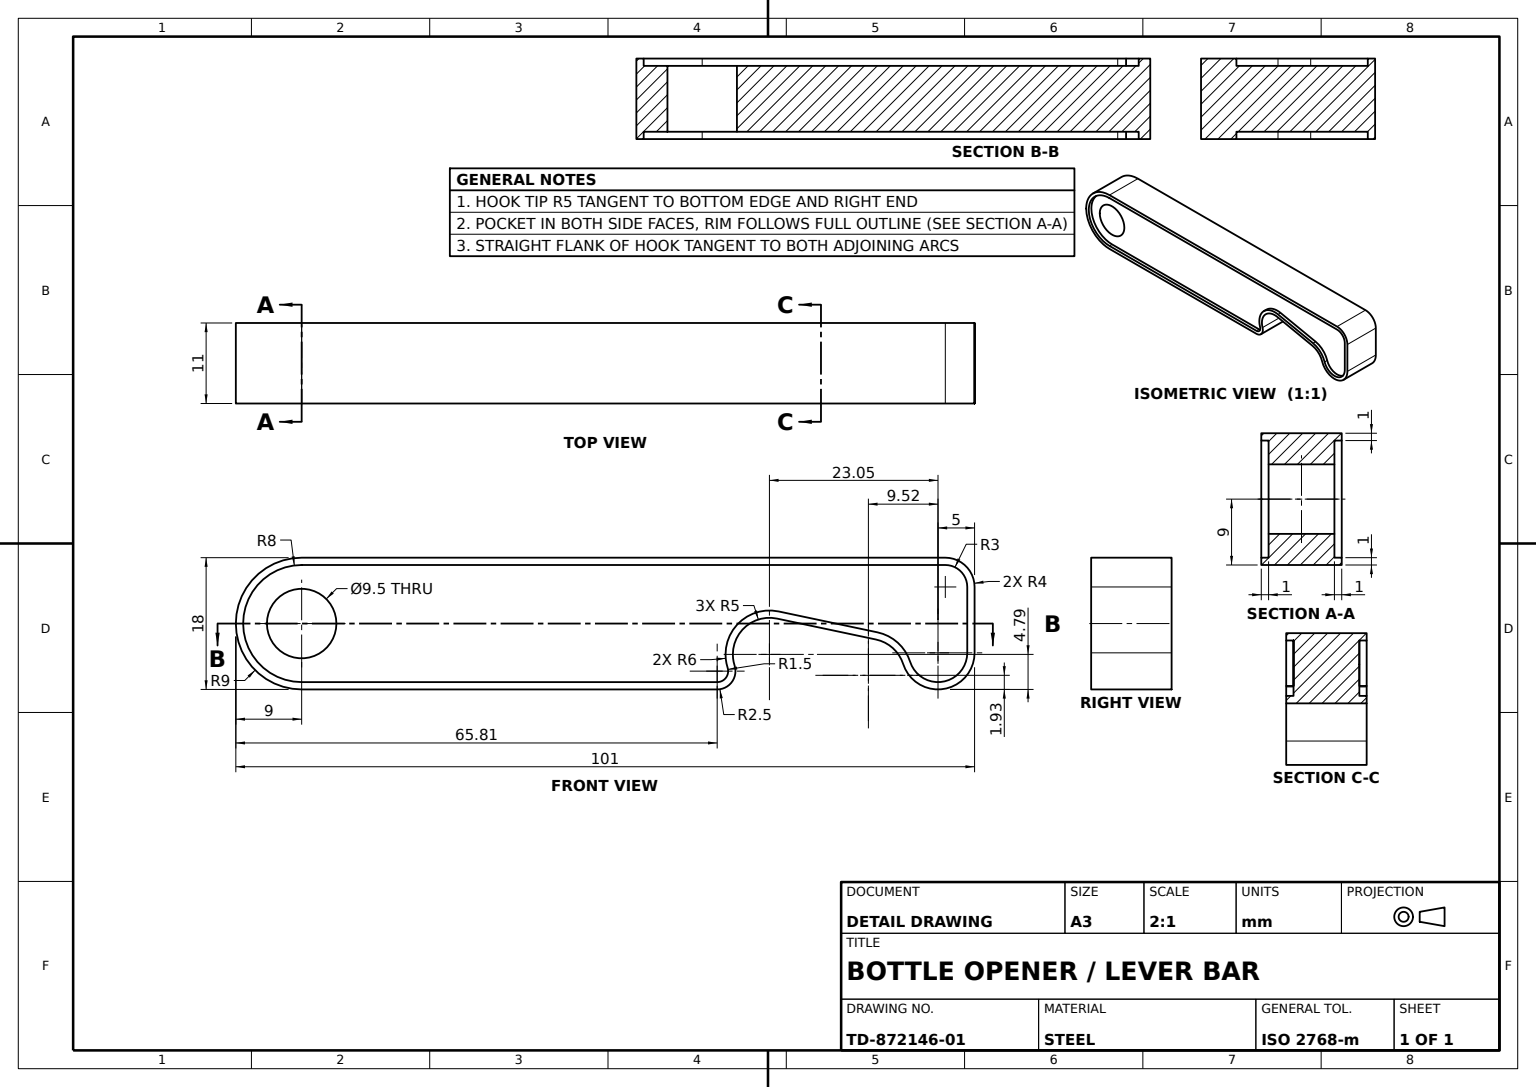
ISO-10303-21;
HEADER;
FILE_DESCRIPTION((''),'2;1');
FILE_NAME('','',(''),(''),'','','');
FILE_SCHEMA(('AUTOMOTIVE_DESIGN'));
ENDSEC;
DATA;
#1=APPLICATION_CONTEXT('');
#2=PRODUCT_CONTEXT('',#1,'mechanical');
#3=PRODUCT('','','',(#2));
#4=PRODUCT_DEFINITION_FORMATION('','',#3);
#5=PRODUCT_DEFINITION_CONTEXT('',#1,'design');
#6=PRODUCT_DEFINITION('','',#4,#5);
#7=PRODUCT_DEFINITION_SHAPE('','',#6);
#8=(LENGTH_UNIT()NAMED_UNIT(*)SI_UNIT(.MILLI.,.METRE.));
#9=(NAMED_UNIT(*)PLANE_ANGLE_UNIT()SI_UNIT($,.RADIAN.));
#10=(NAMED_UNIT(*)SI_UNIT($,.STERADIAN.)SOLID_ANGLE_UNIT());
#11=UNCERTAINTY_MEASURE_WITH_UNIT(LENGTH_MEASURE(1.E-05),#8,'distance_accuracy_value','');
#12=(GEOMETRIC_REPRESENTATION_CONTEXT(3)GLOBAL_UNCERTAINTY_ASSIGNED_CONTEXT((#11))GLOBAL_UNIT_ASSIGNED_CONTEXT((#8,#9,#10))REPRESENTATION_CONTEXT('',''));
#13=CARTESIAN_POINT('',(-9.,0.,5.5));
#14=VERTEX_POINT('',#13);
#15=CARTESIAN_POINT('',(0.,-9.,5.5));
#16=VERTEX_POINT('',#15);
#17=CARTESIAN_POINT('',(0.,0.,5.5));
#18=DIRECTION('',(0.,0.,1.));
#19=DIRECTION('',(1.,0.,0.));
#20=AXIS2_PLACEMENT_3D('',#17,#18,#19);
#21=CIRCLE('',#20,9.);
#22=EDGE_CURVE('',#14,#16,#21,.T.);
#23=ORIENTED_EDGE('',*,*,#22,.F.);
#24=CARTESIAN_POINT('',(-9.,0.,-5.5));
#25=VERTEX_POINT('',#24);
#26=CARTESIAN_POINT('',(-9.,0.,4.5));
#27=DIRECTION('',(0.,0.,-1.));
#28=VECTOR('',#27,1000.);
#29=LINE('',#26,#28);
#30=EDGE_CURVE('',#14,#25,#29,.T.);
#31=ORIENTED_EDGE('',*,*,#30,.T.);
#32=CARTESIAN_POINT('',(0.,-9.,-5.5));
#33=VERTEX_POINT('',#32);
#34=CARTESIAN_POINT('',(0.,0.,-5.5));
#35=AXIS2_PLACEMENT_3D('',#34,#18,#19);
#36=CIRCLE('',#35,9.);
#37=EDGE_CURVE('',#25,#33,#36,.T.);
#38=ORIENTED_EDGE('',*,*,#37,.T.);
#39=CARTESIAN_POINT('',(0.,-9.,4.5));
#40=LINE('',#39,#28);
#41=EDGE_CURVE('',#16,#33,#40,.T.);
#42=ORIENTED_EDGE('',*,*,#41,.F.);
#43=EDGE_LOOP('',(#23,#31,#38,#42));
#44=FACE_OUTER_BOUND('',#43,.T.);
#45=CARTESIAN_POINT('',(0.,0.,4.5));
#46=DIRECTION('',(-1.,0.,0.));
#47=AXIS2_PLACEMENT_3D('',#45,#27,#46);
#48=CYLINDRICAL_SURFACE('',#47,9.);
#49=ADVANCED_FACE('',(#44),#48,.T.);
#50=CARTESIAN_POINT('',(-4.75,0.,4.5));
#51=VERTEX_POINT('',#50);
#52=CARTESIAN_POINT('',(-4.75,0.,-4.5));
#53=VERTEX_POINT('',#52);
#54=CARTESIAN_POINT('',(-4.75,0.,11.5));
#55=LINE('',#54,#28);
#56=EDGE_CURVE('',#51,#53,#55,.T.);
#57=ORIENTED_EDGE('',*,*,#56,.F.);
#58=CARTESIAN_POINT('',(4.75,0.,4.5));
#59=VERTEX_POINT('',#58);
#60=AXIS2_PLACEMENT_3D('',#45,#18,#19);
#61=CIRCLE('',#60,4.75);
#62=EDGE_CURVE('',#51,#59,#61,.T.);
#63=ORIENTED_EDGE('',*,*,#62,.T.);
#64=CARTESIAN_POINT('',(4.75,0.,-4.5));
#65=VERTEX_POINT('',#64);
#66=CARTESIAN_POINT('',(4.75,0.,11.5));
#67=LINE('',#66,#28);
#68=EDGE_CURVE('',#59,#65,#67,.T.);
#69=ORIENTED_EDGE('',*,*,#68,.T.);
#70=CARTESIAN_POINT('',(0.,0.,-4.5));
#71=AXIS2_PLACEMENT_3D('',#70,#27,#46);
#72=CIRCLE('',#71,4.75);
#73=EDGE_CURVE('',#65,#53,#72,.T.);
#74=ORIENTED_EDGE('',*,*,#73,.T.);
#75=EDGE_LOOP('',(#57,#63,#69,#74));
#76=FACE_OUTER_BOUND('',#75,.T.);
#77=CARTESIAN_POINT('',(0.,0.,11.5));
#78=AXIS2_PLACEMENT_3D('',#77,#27,#46);
#79=CYLINDRICAL_SURFACE('',#78,4.75);
#80=ADVANCED_FACE('',(#76),#79,.F.);
#81=CARTESIAN_POINT('',(57.952121,-4.212725,5.5));
#82=VERTEX_POINT('',#81);
#83=CARTESIAN_POINT('',(57.952121,-4.212725,4.5));
#84=VERTEX_POINT('',#83);
#85=LINE('',#81,#28);
#86=EDGE_CURVE('',#82,#84,#85,.T.);
#87=ORIENTED_EDGE('',*,*,#86,.F.);
#88=CARTESIAN_POINT('',(65.192199,1.657727,5.5));
#89=VERTEX_POINT('',#88);
#90=CARTESIAN_POINT('',(63.952121,-4.212725,5.5));
#91=AXIS2_PLACEMENT_3D('',#90,#27,#19);
#92=CIRCLE('',#91,6.);
#93=EDGE_CURVE('',#82,#89,#92,.T.);
#94=ORIENTED_EDGE('',*,*,#93,.T.);
#95=CARTESIAN_POINT('',(65.192199,1.657727,4.5));
#96=VERTEX_POINT('',#95);
#97=LINE('',#88,#28);
#98=EDGE_CURVE('',#89,#96,#97,.T.);
#99=ORIENTED_EDGE('',*,*,#98,.T.);
#100=CARTESIAN_POINT('',(63.952121,-4.212725,4.5));
#101=AXIS2_PLACEMENT_3D('',#100,#27,#19);
#102=CIRCLE('',#101,6.);
#103=EDGE_CURVE('',#84,#96,#102,.T.);
#104=ORIENTED_EDGE('',*,*,#103,.F.);
#105=EDGE_LOOP('',(#87,#94,#99,#104));
#106=FACE_OUTER_BOUND('',#105,.T.);
#107=AXIS2_PLACEMENT_3D('',#90,#27,#46);
#108=CYLINDRICAL_SURFACE('',#107,6.);
#109=ADVANCED_FACE('',(#106),#108,.T.);
#110=CARTESIAN_POINT('',(83.193297,-5.22842,-5.5));
#111=VERTEX_POINT('',#110);
#112=CARTESIAN_POINT('',(91.,-4.,-5.5));
#113=VERTEX_POINT('',#112);
#114=CARTESIAN_POINT('',(87.,-4.,-5.5));
#115=AXIS2_PLACEMENT_3D('',#114,#18,#19);
#116=CIRCLE('',#115,4.);
#117=EDGE_CURVE('',#111,#113,#116,.T.);
#118=ORIENTED_EDGE('',*,*,#117,.F.);
#119=CARTESIAN_POINT('',(83.193297,-5.22842,-4.5));
#120=VERTEX_POINT('',#119);
#121=VECTOR('',#18,1000.);
#122=LINE('',#110,#121);
#123=EDGE_CURVE('',#111,#120,#122,.T.);
#124=ORIENTED_EDGE('',*,*,#123,.T.);
#125=CARTESIAN_POINT('',(91.,-4.,-4.5));
#126=VERTEX_POINT('',#125);
#127=CARTESIAN_POINT('',(87.,-4.,-4.5));
#128=AXIS2_PLACEMENT_3D('',#127,#18,#19);
#129=CIRCLE('',#128,4.);
#130=EDGE_CURVE('',#120,#126,#129,.T.);
#131=ORIENTED_EDGE('',*,*,#130,.T.);
#132=LINE('',#112,#121);
#133=EDGE_CURVE('',#113,#126,#132,.T.);
#134=ORIENTED_EDGE('',*,*,#133,.F.);
#135=EDGE_LOOP('',(#118,#124,#131,#134));
#136=FACE_OUTER_BOUND('',#135,.T.);
#137=CYLINDRICAL_SURFACE('',#115,4.);
#138=ADVANCED_FACE('',(#136),#137,.F.);
#139=CARTESIAN_POINT('',(0.,8.,-5.5));
#140=VERTEX_POINT('',#139);
#141=CARTESIAN_POINT('',(0.,8.,-4.5));
#142=VERTEX_POINT('',#141);
#143=LINE('',#139,#121);
#144=EDGE_CURVE('',#140,#142,#143,.T.);
#145=ORIENTED_EDGE('',*,*,#144,.T.);
#146=CARTESIAN_POINT('',(0.,-8.,-4.5));
#147=VERTEX_POINT('',#146);
#148=AXIS2_PLACEMENT_3D('',#70,#18,#19);
#149=CIRCLE('',#148,8.);
#150=EDGE_CURVE('',#142,#147,#149,.T.);
#151=ORIENTED_EDGE('',*,*,#150,.T.);
#152=CARTESIAN_POINT('',(0.,-8.,-5.5));
#153=VERTEX_POINT('',#152);
#154=LINE('',#152,#121);
#155=EDGE_CURVE('',#153,#147,#154,.T.);
#156=ORIENTED_EDGE('',*,*,#155,.F.);
#157=CIRCLE('',#35,8.);
#158=EDGE_CURVE('',#140,#153,#157,.T.);
#159=ORIENTED_EDGE('',*,*,#158,.F.);
#160=EDGE_LOOP('',(#145,#151,#156,#159));
#161=FACE_OUTER_BOUND('',#160,.T.);
#162=CYLINDRICAL_SURFACE('',#35,8.);
#163=ADVANCED_FACE('',(#161),#162,.F.);
#164=CARTESIAN_POINT('',(58.237949,-6.042545,5.5));
#165=VERTEX_POINT('',#164);
#166=CARTESIAN_POINT('',(58.237949,-6.042545,4.5));
#167=VERTEX_POINT('',#166);
#168=LINE('',#164,#28);
#169=EDGE_CURVE('',#165,#167,#168,.T.);
#170=ORIENTED_EDGE('',*,*,#169,.F.);
#171=EDGE_CURVE('',#165,#82,#92,.T.);
#172=ORIENTED_EDGE('',*,*,#171,.T.);
#173=ORIENTED_EDGE('',*,*,#86,.T.);
#174=EDGE_CURVE('',#167,#84,#102,.T.);
#175=ORIENTED_EDGE('',*,*,#174,.F.);
#176=EDGE_LOOP('',(#170,#172,#173,#175));
#177=FACE_OUTER_BOUND('',#176,.T.);
#178=ADVANCED_FACE('',(#177),#108,.T.);
#179=CARTESIAN_POINT('',(91.,5.,-5.5));
#180=VERTEX_POINT('',#179);
#181=CARTESIAN_POINT('',(91.,5.,-4.5));
#182=VERTEX_POINT('',#181);
#183=LINE('',#179,#121);
#184=EDGE_CURVE('',#180,#182,#183,.T.);
#185=ORIENTED_EDGE('',*,*,#184,.F.);
#186=DIRECTION('',(0.,1.,0.));
#187=VECTOR('',#186,1000.);
#188=LINE('',#112,#187);
#189=EDGE_CURVE('',#113,#180,#188,.T.);
#190=ORIENTED_EDGE('',*,*,#189,.F.);
#191=ORIENTED_EDGE('',*,*,#133,.T.);
#192=LINE('',#125,#187);
#193=EDGE_CURVE('',#126,#182,#192,.T.);
#194=ORIENTED_EDGE('',*,*,#193,.T.);
#195=EDGE_LOOP('',(#185,#190,#191,#194));
#196=FACE_OUTER_BOUND('',#195,.T.);
#197=AXIS2_PLACEMENT_3D('',#112,#19,#27);
#198=PLANE('',#197);
#199=ADVANCED_FACE('',(#196),#198,.F.);
#200=CARTESIAN_POINT('',(56.809406,-8.,-4.5));
#201=VERTEX_POINT('',#200);
#202=CARTESIAN_POINT('',(58.309406,-6.5,-4.5));
#203=VERTEX_POINT('',#202);
#204=CARTESIAN_POINT('',(56.809406,-6.5,-4.5));
#205=AXIS2_PLACEMENT_3D('',#204,#18,#19);
#206=CIRCLE('',#205,1.5);
#207=EDGE_CURVE('',#201,#203,#206,.T.);
#208=ORIENTED_EDGE('',*,*,#207,.T.);
#209=CARTESIAN_POINT('',(58.309406,-6.5,-5.5));
#210=VERTEX_POINT('',#209);
#211=LINE('',#209,#121);
#212=EDGE_CURVE('',#210,#203,#211,.T.);
#213=ORIENTED_EDGE('',*,*,#212,.F.);
#214=CARTESIAN_POINT('',(56.809406,-8.,-5.5));
#215=VERTEX_POINT('',#214);
#216=CARTESIAN_POINT('',(56.809406,-6.5,-5.5));
#217=AXIS2_PLACEMENT_3D('',#216,#18,#19);
#218=CIRCLE('',#217,1.5);
#219=EDGE_CURVE('',#215,#210,#218,.T.);
#220=ORIENTED_EDGE('',*,*,#219,.F.);
#221=LINE('',#214,#121);
#222=EDGE_CURVE('',#215,#201,#221,.T.);
#223=ORIENTED_EDGE('',*,*,#222,.T.);
#224=EDGE_LOOP('',(#208,#213,#220,#223));
#225=FACE_OUTER_BOUND('',#224,.T.);
#226=CYLINDRICAL_SURFACE('',#217,1.5);
#227=ADVANCED_FACE('',(#225),#226,.F.);
#228=CARTESIAN_POINT('',(58.237949,-6.042545,-4.5));
#229=VERTEX_POINT('',#228);
#230=CARTESIAN_POINT('',(65.192199,1.657727,-4.5));
#231=VERTEX_POINT('',#230);
#232=CARTESIAN_POINT('',(63.952121,-4.212725,-4.5));
#233=AXIS2_PLACEMENT_3D('',#232,#27,#19);
#234=CIRCLE('',#233,6.);
#235=EDGE_CURVE('',#229,#231,#234,.T.);
#236=ORIENTED_EDGE('',*,*,#235,.F.);
#237=EDGE_CURVE('',#203,#229,#206,.T.);
#238=ORIENTED_EDGE('',*,*,#237,.F.);
#239=ORIENTED_EDGE('',*,*,#207,.F.);
#240=VECTOR('',#19,1000.);
#241=LINE('',#146,#240);
#242=EDGE_CURVE('',#147,#201,#241,.T.);
#243=ORIENTED_EDGE('',*,*,#242,.F.);
#244=ORIENTED_EDGE('',*,*,#150,.F.);
#245=CARTESIAN_POINT('',(88.,8.,-4.5));
#246=VERTEX_POINT('',#245);
#247=VECTOR('',#46,1000.);
#248=LINE('',#245,#247);
#249=EDGE_CURVE('',#246,#142,#248,.T.);
#250=ORIENTED_EDGE('',*,*,#249,.F.);
#251=CARTESIAN_POINT('',(88.,5.,-4.5));
#252=AXIS2_PLACEMENT_3D('',#251,#18,#19);
#253=CIRCLE('',#252,3.);
#254=EDGE_CURVE('',#182,#246,#253,.T.);
#255=ORIENTED_EDGE('',*,*,#254,.F.);
#256=ORIENTED_EDGE('',*,*,#193,.F.);
#257=ORIENTED_EDGE('',*,*,#130,.F.);
#258=CARTESIAN_POINT('',(78.723322,-1.200598,-4.5));
#259=VERTEX_POINT('',#258);
#260=CARTESIAN_POINT('',(77.483244,-7.07105,-4.5));
#261=AXIS2_PLACEMENT_3D('',#260,#27,#19);
#262=CIRCLE('',#261,6.);
#263=EDGE_CURVE('',#259,#120,#262,.T.);
#264=ORIENTED_EDGE('',*,*,#263,.F.);
#265=DIRECTION('',(0.978408638,-0.206679795,0.));
#266=VECTOR('',#265,1000.);
#267=LINE('',#230,#266);
#268=EDGE_CURVE('',#231,#259,#267,.T.);
#269=ORIENTED_EDGE('',*,*,#268,.F.);
#270=EDGE_LOOP('',(#236,#238,#239,#243,#244,#250,#255,#256,#257,#264,#269));
#271=FACE_OUTER_BOUND('',#270,.T.);
#272=ORIENTED_EDGE('',*,*,#73,.F.);
#273=EDGE_CURVE('',#53,#65,#72,.T.);
#274=ORIENTED_EDGE('',*,*,#273,.F.);
#275=EDGE_LOOP('',(#272,#274));
#276=FACE_BOUND('',#275,.T.);
#277=PLANE('',#148);
#278=ADVANCED_FACE('',(#271,#276),#277,.F.);
#279=CARTESIAN_POINT('',(88.,9.,5.5));
#280=VERTEX_POINT('',#279);
#281=CARTESIAN_POINT('',(88.,9.,-5.5));
#282=VERTEX_POINT('',#281);
#283=CARTESIAN_POINT('',(88.,9.,4.5));
#284=LINE('',#283,#28);
#285=EDGE_CURVE('',#280,#282,#284,.T.);
#286=ORIENTED_EDGE('',*,*,#285,.T.);
#287=CARTESIAN_POINT('',(0.,9.,-5.5));
#288=VERTEX_POINT('',#287);
#289=LINE('',#281,#247);
#290=EDGE_CURVE('',#282,#288,#289,.T.);
#291=ORIENTED_EDGE('',*,*,#290,.T.);
#292=CARTESIAN_POINT('',(0.,9.,5.5));
#293=VERTEX_POINT('',#292);
#294=CARTESIAN_POINT('',(0.,9.,4.5));
#295=LINE('',#294,#28);
#296=EDGE_CURVE('',#293,#288,#295,.T.);
#297=ORIENTED_EDGE('',*,*,#296,.F.);
#298=LINE('',#279,#247);
#299=EDGE_CURVE('',#280,#293,#298,.T.);
#300=ORIENTED_EDGE('',*,*,#299,.F.);
#301=EDGE_LOOP('',(#286,#291,#297,#300));
#302=FACE_OUTER_BOUND('',#301,.T.);
#303=AXIS2_PLACEMENT_3D('',#294,#186,#18);
#304=PLANE('',#303);
#305=ADVANCED_FACE('',(#302),#304,.T.);
#306=CARTESIAN_POINT('',(56.809406,-8.,5.5));
#307=VERTEX_POINT('',#306);
#308=CARTESIAN_POINT('',(56.809406,-8.,4.5));
#309=VERTEX_POINT('',#308);
#310=LINE('',#306,#28);
#311=EDGE_CURVE('',#307,#309,#310,.T.);
#312=ORIENTED_EDGE('',*,*,#311,.F.);
#313=CARTESIAN_POINT('',(56.809406,-6.5,5.5));
#314=AXIS2_PLACEMENT_3D('',#313,#18,#19);
#315=CIRCLE('',#314,1.5);
#316=EDGE_CURVE('',#307,#165,#315,.T.);
#317=ORIENTED_EDGE('',*,*,#316,.T.);
#318=ORIENTED_EDGE('',*,*,#169,.T.);
#319=CARTESIAN_POINT('',(56.809406,-6.5,4.5));
#320=AXIS2_PLACEMENT_3D('',#319,#18,#19);
#321=CIRCLE('',#320,1.5);
#322=EDGE_CURVE('',#309,#167,#321,.T.);
#323=ORIENTED_EDGE('',*,*,#322,.F.);
#324=EDGE_LOOP('',(#312,#317,#318,#323));
#325=FACE_OUTER_BOUND('',#324,.T.);
#326=AXIS2_PLACEMENT_3D('',#313,#27,#46);
#327=CYLINDRICAL_SURFACE('',#326,1.5);
#328=ADVANCED_FACE('',(#325),#327,.F.);
#329=CARTESIAN_POINT('',(64.98552,0.679318,5.5));
#330=VERTEX_POINT('',#329);
#331=CARTESIAN_POINT('',(64.98552,0.679318,-5.5));
#332=VERTEX_POINT('',#331);
#333=CARTESIAN_POINT('',(64.98552,0.679318,4.5));
#334=LINE('',#333,#28);
#335=EDGE_CURVE('',#330,#332,#334,.T.);
#336=ORIENTED_EDGE('',*,*,#335,.F.);
#337=CARTESIAN_POINT('',(58.952121,-4.212725,5.5));
#338=VERTEX_POINT('',#337);
#339=CIRCLE('',#91,5.);
#340=EDGE_CURVE('',#338,#330,#339,.T.);
#341=ORIENTED_EDGE('',*,*,#340,.F.);
#342=CARTESIAN_POINT('',(58.952121,-4.212725,-5.5));
#343=VERTEX_POINT('',#342);
#344=CARTESIAN_POINT('',(58.952121,-4.212725,4.5));
#345=LINE('',#344,#28);
#346=EDGE_CURVE('',#338,#343,#345,.T.);
#347=ORIENTED_EDGE('',*,*,#346,.T.);
#348=CARTESIAN_POINT('',(63.952121,-4.212725,-5.5));
#349=AXIS2_PLACEMENT_3D('',#348,#27,#19);
#350=CIRCLE('',#349,5.);
#351=EDGE_CURVE('',#343,#332,#350,.T.);
#352=ORIENTED_EDGE('',*,*,#351,.T.);
#353=EDGE_LOOP('',(#336,#341,#347,#352));
#354=FACE_OUTER_BOUND('',#353,.T.);
#355=AXIS2_PLACEMENT_3D('',#100,#27,#46);
#356=CYLINDRICAL_SURFACE('',#355,5.);
#357=ADVANCED_FACE('',(#354),#356,.F.);
#358=CARTESIAN_POINT('',(0.,8.,5.5));
#359=VERTEX_POINT('',#358);
#360=CARTESIAN_POINT('',(0.,8.,4.5));
#361=VERTEX_POINT('',#360);
#362=LINE('',#358,#28);
#363=EDGE_CURVE('',#359,#361,#362,.T.);
#364=ORIENTED_EDGE('',*,*,#363,.F.);
#365=CARTESIAN_POINT('',(-8.,0.,5.5));
#366=VERTEX_POINT('',#365);
#367=CIRCLE('',#20,8.);
#368=EDGE_CURVE('',#359,#366,#367,.T.);
#369=ORIENTED_EDGE('',*,*,#368,.T.);
#370=CARTESIAN_POINT('',(-8.,0.,4.5));
#371=VERTEX_POINT('',#370);
#372=LINE('',#365,#28);
#373=EDGE_CURVE('',#366,#371,#372,.T.);
#374=ORIENTED_EDGE('',*,*,#373,.T.);
#375=CIRCLE('',#60,8.);
#376=EDGE_CURVE('',#361,#371,#375,.T.);
#377=ORIENTED_EDGE('',*,*,#376,.F.);
#378=EDGE_LOOP('',(#364,#369,#374,#377));
#379=FACE_OUTER_BOUND('',#378,.T.);
#380=AXIS2_PLACEMENT_3D('',#17,#27,#46);
#381=CYLINDRICAL_SURFACE('',#380,8.);
#382=ADVANCED_FACE('',(#379),#381,.F.);
#383=CARTESIAN_POINT('',(59.190311,-5.737575,-5.5));
#384=VERTEX_POINT('',#383);
#385=EDGE_CURVE('',#384,#343,#350,.T.);
#386=ORIENTED_EDGE('',*,*,#385,.T.);
#387=ORIENTED_EDGE('',*,*,#346,.F.);
#388=CARTESIAN_POINT('',(59.190311,-5.737575,5.5));
#389=VERTEX_POINT('',#388);
#390=EDGE_CURVE('',#389,#338,#339,.T.);
#391=ORIENTED_EDGE('',*,*,#390,.F.);
#392=CARTESIAN_POINT('',(59.190311,-5.737575,4.5));
#393=LINE('',#392,#28);
#394=EDGE_CURVE('',#389,#384,#393,.T.);
#395=ORIENTED_EDGE('',*,*,#394,.T.);
#396=EDGE_LOOP('',(#386,#387,#391,#395));
#397=FACE_OUTER_BOUND('',#396,.T.);
#398=ADVANCED_FACE('',(#397),#356,.F.);
#399=CARTESIAN_POINT('',(58.237949,-6.042545,-5.5));
#400=VERTEX_POINT('',#399);
#401=CARTESIAN_POINT('',(65.192199,1.657727,-5.5));
#402=VERTEX_POINT('',#401);
#403=CIRCLE('',#349,6.);
#404=EDGE_CURVE('',#400,#402,#403,.T.);
#405=ORIENTED_EDGE('',*,*,#404,.F.);
#406=LINE('',#399,#121);
#407=EDGE_CURVE('',#400,#229,#406,.T.);
#408=ORIENTED_EDGE('',*,*,#407,.T.);
#409=ORIENTED_EDGE('',*,*,#235,.T.);
#410=LINE('',#401,#121);
#411=EDGE_CURVE('',#402,#231,#410,.T.);
#412=ORIENTED_EDGE('',*,*,#411,.F.);
#413=EDGE_LOOP('',(#405,#408,#409,#412));
#414=FACE_OUTER_BOUND('',#413,.T.);
#415=AXIS2_PLACEMENT_3D('',#348,#18,#19);
#416=CYLINDRICAL_SURFACE('',#415,6.);
#417=ADVANCED_FACE('',(#414),#416,.T.);
#418=ORIENTED_EDGE('',*,*,#407,.F.);
#419=EDGE_CURVE('',#210,#400,#218,.T.);
#420=ORIENTED_EDGE('',*,*,#419,.F.);
#421=ORIENTED_EDGE('',*,*,#212,.T.);
#422=ORIENTED_EDGE('',*,*,#237,.T.);
#423=EDGE_LOOP('',(#418,#420,#421,#422));
#424=FACE_OUTER_BOUND('',#423,.T.);
#425=ADVANCED_FACE('',(#424),#226,.F.);
#426=CARTESIAN_POINT('',(82.241622,-5.535525,5.5));
#427=VERTEX_POINT('',#426);
#428=CARTESIAN_POINT('',(82.241622,-5.535525,-5.5));
#429=VERTEX_POINT('',#428);
#430=CARTESIAN_POINT('',(82.241622,-5.535525,4.5));
#431=LINE('',#430,#28);
#432=EDGE_CURVE('',#427,#429,#431,.T.);
#433=ORIENTED_EDGE('',*,*,#432,.T.);
#434=CARTESIAN_POINT('',(92.,-4.,-5.5));
#435=VERTEX_POINT('',#434);
#436=CIRCLE('',#115,5.);
#437=EDGE_CURVE('',#429,#435,#436,.T.);
#438=ORIENTED_EDGE('',*,*,#437,.T.);
#439=CARTESIAN_POINT('',(92.,-4.,5.5));
#440=VERTEX_POINT('',#439);
#441=CARTESIAN_POINT('',(92.,-4.,4.5));
#442=LINE('',#441,#28);
#443=EDGE_CURVE('',#440,#435,#442,.T.);
#444=ORIENTED_EDGE('',*,*,#443,.F.);
#445=CARTESIAN_POINT('',(87.,-4.,5.5));
#446=AXIS2_PLACEMENT_3D('',#445,#18,#19);
#447=CIRCLE('',#446,5.);
#448=EDGE_CURVE('',#427,#440,#447,.T.);
#449=ORIENTED_EDGE('',*,*,#448,.F.);
#450=EDGE_LOOP('',(#433,#438,#444,#449));
#451=FACE_OUTER_BOUND('',#450,.T.);
#452=CARTESIAN_POINT('',(87.,-4.,4.5));
#453=AXIS2_PLACEMENT_3D('',#452,#27,#46);
#454=CYLINDRICAL_SURFACE('',#453,5.);
#455=ADVANCED_FACE('',(#451),#454,.T.);
#456=ORIENTED_EDGE('',*,*,#249,.T.);
#457=ORIENTED_EDGE('',*,*,#144,.F.);
#458=CARTESIAN_POINT('',(88.,8.,-5.5));
#459=VERTEX_POINT('',#458);
#460=LINE('',#458,#247);
#461=EDGE_CURVE('',#459,#140,#460,.T.);
#462=ORIENTED_EDGE('',*,*,#461,.F.);
#463=LINE('',#458,#121);
#464=EDGE_CURVE('',#459,#246,#463,.T.);
#465=ORIENTED_EDGE('',*,*,#464,.T.);
#466=EDGE_LOOP('',(#456,#457,#462,#465));
#467=FACE_OUTER_BOUND('',#466,.T.);
#468=AXIS2_PLACEMENT_3D('',#458,#186,#46);
#469=PLANE('',#468);
#470=ADVANCED_FACE('',(#467),#469,.F.);
#471=CARTESIAN_POINT('',(78.723322,-1.200598,-5.5));
#472=VERTEX_POINT('',#471);
#473=LINE('',#401,#266);
#474=EDGE_CURVE('',#402,#472,#473,.T.);
#475=ORIENTED_EDGE('',*,*,#474,.F.);
#476=ORIENTED_EDGE('',*,*,#411,.T.);
#477=ORIENTED_EDGE('',*,*,#268,.T.);
#478=LINE('',#471,#121);
#479=EDGE_CURVE('',#472,#259,#478,.T.);
#480=ORIENTED_EDGE('',*,*,#479,.F.);
#481=EDGE_LOOP('',(#475,#476,#477,#480));
#482=FACE_OUTER_BOUND('',#481,.T.);
#483=DIRECTION('',(-0.206679795,-0.978408638,0.));
#484=AXIS2_PLACEMENT_3D('',#401,#483,#265);
#485=PLANE('',#484);
#486=ADVANCED_FACE('',(#482),#485,.F.);
#487=CARTESIAN_POINT('',(83.193297,-5.22842,5.5));
#488=VERTEX_POINT('',#487);
#489=CARTESIAN_POINT('',(91.,-4.,5.5));
#490=VERTEX_POINT('',#489);
#491=CIRCLE('',#446,4.);
#492=EDGE_CURVE('',#488,#490,#491,.T.);
#493=ORIENTED_EDGE('',*,*,#492,.T.);
#494=CARTESIAN_POINT('',(91.,-4.,4.5));
#495=VERTEX_POINT('',#494);
#496=LINE('',#489,#28);
#497=EDGE_CURVE('',#490,#495,#496,.T.);
#498=ORIENTED_EDGE('',*,*,#497,.T.);
#499=CARTESIAN_POINT('',(83.193297,-5.22842,4.5));
#500=VERTEX_POINT('',#499);
#501=AXIS2_PLACEMENT_3D('',#452,#18,#19);
#502=CIRCLE('',#501,4.);
#503=EDGE_CURVE('',#500,#495,#502,.T.);
#504=ORIENTED_EDGE('',*,*,#503,.F.);
#505=LINE('',#487,#28);
#506=EDGE_CURVE('',#488,#500,#505,.T.);
#507=ORIENTED_EDGE('',*,*,#506,.F.);
#508=EDGE_LOOP('',(#493,#498,#504,#507));
#509=FACE_OUTER_BOUND('',#508,.T.);
#510=AXIS2_PLACEMENT_3D('',#445,#27,#46);
#511=CYLINDRICAL_SURFACE('',#510,4.);
#512=ADVANCED_FACE('',(#509),#511,.F.);
#513=ORIENTED_EDGE('',*,*,#322,.T.);
#514=ORIENTED_EDGE('',*,*,#174,.T.);
#515=ORIENTED_EDGE('',*,*,#103,.T.);
#516=CARTESIAN_POINT('',(78.723322,-1.200598,4.5));
#517=VERTEX_POINT('',#516);
#518=LINE('',#95,#266);
#519=EDGE_CURVE('',#96,#517,#518,.T.);
#520=ORIENTED_EDGE('',*,*,#519,.T.);
#521=CARTESIAN_POINT('',(77.483244,-7.07105,4.5));
#522=AXIS2_PLACEMENT_3D('',#521,#27,#19);
#523=CIRCLE('',#522,6.);
#524=EDGE_CURVE('',#517,#500,#523,.T.);
#525=ORIENTED_EDGE('',*,*,#524,.T.);
#526=ORIENTED_EDGE('',*,*,#503,.T.);
#527=CARTESIAN_POINT('',(91.,5.,4.5));
#528=VERTEX_POINT('',#527);
#529=LINE('',#494,#187);
#530=EDGE_CURVE('',#495,#528,#529,.T.);
#531=ORIENTED_EDGE('',*,*,#530,.T.);
#532=CARTESIAN_POINT('',(88.,8.,4.5));
#533=VERTEX_POINT('',#532);
#534=CARTESIAN_POINT('',(88.,5.,4.5));
#535=AXIS2_PLACEMENT_3D('',#534,#18,#19);
#536=CIRCLE('',#535,3.);
#537=EDGE_CURVE('',#528,#533,#536,.T.);
#538=ORIENTED_EDGE('',*,*,#537,.T.);
#539=LINE('',#532,#247);
#540=EDGE_CURVE('',#533,#361,#539,.T.);
#541=ORIENTED_EDGE('',*,*,#540,.T.);
#542=ORIENTED_EDGE('',*,*,#376,.T.);
#543=CARTESIAN_POINT('',(0.,-8.,4.5));
#544=VERTEX_POINT('',#543);
#545=EDGE_CURVE('',#371,#544,#375,.T.);
#546=ORIENTED_EDGE('',*,*,#545,.T.);
#547=LINE('',#543,#240);
#548=EDGE_CURVE('',#544,#309,#547,.T.);
#549=ORIENTED_EDGE('',*,*,#548,.T.);
#550=EDGE_LOOP('',(#513,#514,#515,#520,#525,#526,#531,#538,#541,#542,#546,#549));
#551=FACE_OUTER_BOUND('',#550,.T.);
#552=ORIENTED_EDGE('',*,*,#62,.F.);
#553=EDGE_CURVE('',#59,#51,#61,.T.);
#554=ORIENTED_EDGE('',*,*,#553,.F.);
#555=EDGE_LOOP('',(#552,#554));
#556=FACE_BOUND('',#555,.T.);
#557=PLANE('',#60);
#558=ADVANCED_FACE('',(#551,#556),#557,.T.);
#559=CARTESIAN_POINT('',(92.,5.,5.5));
#560=VERTEX_POINT('',#559);
#561=CARTESIAN_POINT('',(92.,5.,-5.5));
#562=VERTEX_POINT('',#561);
#563=CARTESIAN_POINT('',(92.,5.,4.5));
#564=LINE('',#563,#28);
#565=EDGE_CURVE('',#560,#562,#564,.T.);
#566=ORIENTED_EDGE('',*,*,#565,.F.);
#567=LINE('',#439,#187);
#568=EDGE_CURVE('',#440,#560,#567,.T.);
#569=ORIENTED_EDGE('',*,*,#568,.F.);
#570=ORIENTED_EDGE('',*,*,#443,.T.);
#571=LINE('',#434,#187);
#572=EDGE_CURVE('',#435,#562,#571,.T.);
#573=ORIENTED_EDGE('',*,*,#572,.T.);
#574=EDGE_LOOP('',(#566,#569,#570,#573));
#575=FACE_OUTER_BOUND('',#574,.T.);
#576=CARTESIAN_POINT('',(92.,0.,4.5));
#577=AXIS2_PLACEMENT_3D('',#576,#19,#186);
#578=PLANE('',#577);
#579=ADVANCED_FACE('',(#575),#578,.T.);
#580=ORIENTED_EDGE('',*,*,#540,.F.);
#581=CARTESIAN_POINT('',(88.,8.,5.5));
#582=VERTEX_POINT('',#581);
#583=LINE('',#581,#28);
#584=EDGE_CURVE('',#582,#533,#583,.T.);
#585=ORIENTED_EDGE('',*,*,#584,.F.);
#586=LINE('',#581,#247);
#587=EDGE_CURVE('',#582,#359,#586,.T.);
#588=ORIENTED_EDGE('',*,*,#587,.T.);
#589=ORIENTED_EDGE('',*,*,#363,.T.);
#590=EDGE_LOOP('',(#580,#585,#588,#589));
#591=FACE_OUTER_BOUND('',#590,.T.);
#592=DIRECTION('',(0.,-1.,0.));
#593=AXIS2_PLACEMENT_3D('',#581,#592,#19);
#594=PLANE('',#593);
#595=ADVANCED_FACE('',(#591),#594,.T.);
#596=LINE('',#152,#240);
#597=EDGE_CURVE('',#153,#215,#596,.T.);
#598=ORIENTED_EDGE('',*,*,#597,.F.);
#599=ORIENTED_EDGE('',*,*,#155,.T.);
#600=ORIENTED_EDGE('',*,*,#242,.T.);
#601=ORIENTED_EDGE('',*,*,#222,.F.);
#602=EDGE_LOOP('',(#598,#599,#600,#601));
#603=FACE_OUTER_BOUND('',#602,.T.);
#604=AXIS2_PLACEMENT_3D('',#152,#592,#27);
#605=PLANE('',#604);
#606=ADVANCED_FACE('',(#603),#605,.F.);
#607=CARTESIAN_POINT('',(56.809406,-9.,-5.5));
#608=VERTEX_POINT('',#607);
#609=CIRCLE('',#217,2.5);
#610=EDGE_CURVE('',#608,#384,#609,.T.);
#611=ORIENTED_EDGE('',*,*,#610,.T.);
#612=ORIENTED_EDGE('',*,*,#394,.F.);
#613=CARTESIAN_POINT('',(56.809406,-9.,5.5));
#614=VERTEX_POINT('',#613);
#615=CIRCLE('',#314,2.5);
#616=EDGE_CURVE('',#614,#389,#615,.T.);
#617=ORIENTED_EDGE('',*,*,#616,.F.);
#618=CARTESIAN_POINT('',(56.809406,-9.,4.5));
#619=LINE('',#618,#28);
#620=EDGE_CURVE('',#614,#608,#619,.T.);
#621=ORIENTED_EDGE('',*,*,#620,.T.);
#622=EDGE_LOOP('',(#611,#612,#617,#621));
#623=FACE_OUTER_BOUND('',#622,.T.);
#624=AXIS2_PLACEMENT_3D('',#319,#27,#46);
#625=CYLINDRICAL_SURFACE('',#624,2.5);
#626=ADVANCED_FACE('',(#623),#625,.T.);
#627=ORIENTED_EDGE('',*,*,#519,.F.);
#628=ORIENTED_EDGE('',*,*,#98,.F.);
#629=CARTESIAN_POINT('',(78.723322,-1.200598,5.5));
#630=VERTEX_POINT('',#629);
#631=LINE('',#88,#266);
#632=EDGE_CURVE('',#89,#630,#631,.T.);
#633=ORIENTED_EDGE('',*,*,#632,.T.);
#634=LINE('',#629,#28);
#635=EDGE_CURVE('',#630,#517,#634,.T.);
#636=ORIENTED_EDGE('',*,*,#635,.T.);
#637=EDGE_LOOP('',(#627,#628,#633,#636));
#638=FACE_OUTER_BOUND('',#637,.T.);
#639=DIRECTION('',(0.206679795,0.978408638,0.));
#640=DIRECTION('',(-0.978408638,0.206679795,0.));
#641=AXIS2_PLACEMENT_3D('',#88,#639,#640);
#642=PLANE('',#641);
#643=ADVANCED_FACE('',(#638),#642,.T.);
#644=ORIENTED_EDGE('',*,*,#548,.F.);
#645=CARTESIAN_POINT('',(0.,-8.,5.5));
#646=VERTEX_POINT('',#645);
#647=LINE('',#645,#28);
#648=EDGE_CURVE('',#646,#544,#647,.T.);
#649=ORIENTED_EDGE('',*,*,#648,.F.);
#650=LINE('',#645,#240);
#651=EDGE_CURVE('',#646,#307,#650,.T.);
#652=ORIENTED_EDGE('',*,*,#651,.T.);
#653=ORIENTED_EDGE('',*,*,#311,.T.);
#654=EDGE_LOOP('',(#644,#649,#652,#653));
#655=FACE_OUTER_BOUND('',#654,.T.);
#656=AXIS2_PLACEMENT_3D('',#645,#186,#18);
#657=PLANE('',#656);
#658=ADVANCED_FACE('',(#655),#657,.T.);
#659=CARTESIAN_POINT('',(91.,5.,5.5));
#660=VERTEX_POINT('',#659);
#661=CARTESIAN_POINT('',(88.,5.,5.5));
#662=AXIS2_PLACEMENT_3D('',#661,#18,#19);
#663=CIRCLE('',#662,3.);
#664=EDGE_CURVE('',#660,#582,#663,.T.);
#665=ORIENTED_EDGE('',*,*,#664,.T.);
#666=ORIENTED_EDGE('',*,*,#584,.T.);
#667=ORIENTED_EDGE('',*,*,#537,.F.);
#668=LINE('',#659,#28);
#669=EDGE_CURVE('',#660,#528,#668,.T.);
#670=ORIENTED_EDGE('',*,*,#669,.F.);
#671=EDGE_LOOP('',(#665,#666,#667,#670));
#672=FACE_OUTER_BOUND('',#671,.T.);
#673=AXIS2_PLACEMENT_3D('',#661,#27,#46);
#674=CYLINDRICAL_SURFACE('',#673,3.);
#675=ADVANCED_FACE('',(#672),#674,.F.);
#676=EDGE_CURVE('',#293,#14,#21,.T.);
#677=ORIENTED_EDGE('',*,*,#676,.F.);
#678=ORIENTED_EDGE('',*,*,#296,.T.);
#679=EDGE_CURVE('',#288,#25,#36,.T.);
#680=ORIENTED_EDGE('',*,*,#679,.T.);
#681=ORIENTED_EDGE('',*,*,#30,.F.);
#682=EDGE_LOOP('',(#677,#678,#680,#681));
#683=FACE_OUTER_BOUND('',#682,.T.);
#684=ADVANCED_FACE('',(#683),#48,.T.);
#685=ORIENTED_EDGE('',*,*,#117,.T.);
#686=ORIENTED_EDGE('',*,*,#189,.T.);
#687=CARTESIAN_POINT('',(88.,5.,-5.5));
#688=AXIS2_PLACEMENT_3D('',#687,#18,#19);
#689=CIRCLE('',#688,3.);
#690=EDGE_CURVE('',#180,#459,#689,.T.);
#691=ORIENTED_EDGE('',*,*,#690,.T.);
#692=ORIENTED_EDGE('',*,*,#461,.T.);
#693=ORIENTED_EDGE('',*,*,#158,.T.);
#694=ORIENTED_EDGE('',*,*,#597,.T.);
#695=ORIENTED_EDGE('',*,*,#219,.T.);
#696=ORIENTED_EDGE('',*,*,#419,.T.);
#697=ORIENTED_EDGE('',*,*,#404,.T.);
#698=ORIENTED_EDGE('',*,*,#474,.T.);
#699=CARTESIAN_POINT('',(77.483244,-7.07105,-5.5));
#700=AXIS2_PLACEMENT_3D('',#699,#27,#19);
#701=CIRCLE('',#700,6.);
#702=EDGE_CURVE('',#472,#111,#701,.T.);
#703=ORIENTED_EDGE('',*,*,#702,.T.);
#704=EDGE_LOOP('',(#685,#686,#691,#692,#693,#694,#695,#696,#697,#698,#703));
#705=FACE_BOUND('',#704,.T.);
#706=CARTESIAN_POINT('',(78.516643,-2.179007,-5.5));
#707=VERTEX_POINT('',#706);
#708=LINE('',#331,#266);
#709=EDGE_CURVE('',#332,#707,#708,.T.);
#710=ORIENTED_EDGE('',*,*,#709,.F.);
#711=ORIENTED_EDGE('',*,*,#351,.F.);
#712=ORIENTED_EDGE('',*,*,#385,.F.);
#713=ORIENTED_EDGE('',*,*,#610,.F.);
#714=LINE('',#32,#240);
#715=EDGE_CURVE('',#33,#608,#714,.T.);
#716=ORIENTED_EDGE('',*,*,#715,.F.);
#717=ORIENTED_EDGE('',*,*,#37,.F.);
#718=ORIENTED_EDGE('',*,*,#679,.F.);
#719=ORIENTED_EDGE('',*,*,#290,.F.);
#720=CIRCLE('',#688,4.);
#721=EDGE_CURVE('',#562,#282,#720,.T.);
#722=ORIENTED_EDGE('',*,*,#721,.F.);
#723=ORIENTED_EDGE('',*,*,#572,.F.);
#724=ORIENTED_EDGE('',*,*,#437,.F.);
#725=CIRCLE('',#700,5.);
#726=EDGE_CURVE('',#707,#429,#725,.T.);
#727=ORIENTED_EDGE('',*,*,#726,.F.);
#728=EDGE_LOOP('',(#710,#711,#712,#713,#716,#717,#718,#719,#722,#723,#724,#727));
#729=FACE_OUTER_BOUND('',#728,.T.);
#730=AXIS2_PLACEMENT_3D('',#216,#27,#19);
#731=PLANE('',#730);
#732=ADVANCED_FACE('',(#705,#729),#731,.T.);
#733=ORIENTED_EDGE('',*,*,#721,.T.);
#734=ORIENTED_EDGE('',*,*,#285,.F.);
#735=CIRCLE('',#662,4.);
#736=EDGE_CURVE('',#560,#280,#735,.T.);
#737=ORIENTED_EDGE('',*,*,#736,.F.);
#738=ORIENTED_EDGE('',*,*,#565,.T.);
#739=EDGE_LOOP('',(#733,#734,#737,#738));
#740=FACE_OUTER_BOUND('',#739,.T.);
#741=AXIS2_PLACEMENT_3D('',#534,#27,#46);
#742=CYLINDRICAL_SURFACE('',#741,4.);
#743=ADVANCED_FACE('',(#740),#742,.T.);
#744=ORIENTED_EDGE('',*,*,#56,.T.);
#745=ORIENTED_EDGE('',*,*,#273,.T.);
#746=ORIENTED_EDGE('',*,*,#68,.F.);
#747=ORIENTED_EDGE('',*,*,#553,.T.);
#748=EDGE_LOOP('',(#744,#745,#746,#747));
#749=FACE_OUTER_BOUND('',#748,.T.);
#750=ADVANCED_FACE('',(#749),#79,.F.);
#751=CARTESIAN_POINT('',(78.516643,-2.179007,5.5));
#752=VERTEX_POINT('',#751);
#753=LINE('',#329,#266);
#754=EDGE_CURVE('',#330,#752,#753,.T.);
#755=ORIENTED_EDGE('',*,*,#754,.F.);
#756=ORIENTED_EDGE('',*,*,#335,.T.);
#757=ORIENTED_EDGE('',*,*,#709,.T.);
#758=CARTESIAN_POINT('',(78.516643,-2.179007,4.5));
#759=LINE('',#758,#28);
#760=EDGE_CURVE('',#752,#707,#759,.T.);
#761=ORIENTED_EDGE('',*,*,#760,.F.);
#762=EDGE_LOOP('',(#755,#756,#757,#761));
#763=FACE_OUTER_BOUND('',#762,.T.);
#764=CARTESIAN_POINT('',(2.913326,13.791496,4.5));
#765=AXIS2_PLACEMENT_3D('',#764,#639,#640);
#766=PLANE('',#765);
#767=ADVANCED_FACE('',(#763),#766,.F.);
#768=CARTESIAN_POINT('',(77.483244,-7.07105,5.5));
#769=AXIS2_PLACEMENT_3D('',#768,#27,#19);
#770=CIRCLE('',#769,6.);
#771=EDGE_CURVE('',#630,#488,#770,.T.);
#772=ORIENTED_EDGE('',*,*,#771,.T.);
#773=ORIENTED_EDGE('',*,*,#506,.T.);
#774=ORIENTED_EDGE('',*,*,#524,.F.);
#775=ORIENTED_EDGE('',*,*,#635,.F.);
#776=EDGE_LOOP('',(#772,#773,#774,#775));
#777=FACE_OUTER_BOUND('',#776,.T.);
#778=AXIS2_PLACEMENT_3D('',#768,#27,#46);
#779=CYLINDRICAL_SURFACE('',#778,6.);
#780=ADVANCED_FACE('',(#777),#779,.T.);
#781=ORIENTED_EDGE('',*,*,#41,.T.);
#782=ORIENTED_EDGE('',*,*,#715,.T.);
#783=ORIENTED_EDGE('',*,*,#620,.F.);
#784=LINE('',#15,#240);
#785=EDGE_CURVE('',#16,#614,#784,.T.);
#786=ORIENTED_EDGE('',*,*,#785,.F.);
#787=EDGE_LOOP('',(#781,#782,#783,#786));
#788=FACE_OUTER_BOUND('',#787,.T.);
#789=AXIS2_PLACEMENT_3D('',#39,#186,#46);
#790=PLANE('',#789);
#791=ADVANCED_FACE('',(#788),#790,.F.);
#792=EDGE_CURVE('',#366,#646,#367,.T.);
#793=ORIENTED_EDGE('',*,*,#792,.T.);
#794=ORIENTED_EDGE('',*,*,#648,.T.);
#795=ORIENTED_EDGE('',*,*,#545,.F.);
#796=ORIENTED_EDGE('',*,*,#373,.F.);
#797=EDGE_LOOP('',(#793,#794,#795,#796));
#798=FACE_OUTER_BOUND('',#797,.T.);
#799=ADVANCED_FACE('',(#798),#381,.F.);
#800=ORIENTED_EDGE('',*,*,#785,.T.);
#801=ORIENTED_EDGE('',*,*,#616,.T.);
#802=ORIENTED_EDGE('',*,*,#390,.T.);
#803=ORIENTED_EDGE('',*,*,#340,.T.);
#804=ORIENTED_EDGE('',*,*,#754,.T.);
#805=CIRCLE('',#769,5.);
#806=EDGE_CURVE('',#752,#427,#805,.T.);
#807=ORIENTED_EDGE('',*,*,#806,.T.);
#808=ORIENTED_EDGE('',*,*,#448,.T.);
#809=ORIENTED_EDGE('',*,*,#568,.T.);
#810=ORIENTED_EDGE('',*,*,#736,.T.);
#811=ORIENTED_EDGE('',*,*,#299,.T.);
#812=ORIENTED_EDGE('',*,*,#676,.T.);
#813=ORIENTED_EDGE('',*,*,#22,.T.);
#814=EDGE_LOOP('',(#800,#801,#802,#803,#804,#807,#808,#809,#810,#811,#812,#813));
#815=FACE_OUTER_BOUND('',#814,.T.);
#816=ORIENTED_EDGE('',*,*,#587,.F.);
#817=ORIENTED_EDGE('',*,*,#664,.F.);
#818=LINE('',#489,#187);
#819=EDGE_CURVE('',#490,#660,#818,.T.);
#820=ORIENTED_EDGE('',*,*,#819,.F.);
#821=ORIENTED_EDGE('',*,*,#492,.F.);
#822=ORIENTED_EDGE('',*,*,#771,.F.);
#823=ORIENTED_EDGE('',*,*,#632,.F.);
#824=ORIENTED_EDGE('',*,*,#93,.F.);
#825=ORIENTED_EDGE('',*,*,#171,.F.);
#826=ORIENTED_EDGE('',*,*,#316,.F.);
#827=ORIENTED_EDGE('',*,*,#651,.F.);
#828=ORIENTED_EDGE('',*,*,#792,.F.);
#829=ORIENTED_EDGE('',*,*,#368,.F.);
#830=EDGE_LOOP('',(#816,#817,#820,#821,#822,#823,#824,#825,#826,#827,#828,#829));
#831=FACE_BOUND('',#830,.T.);
#832=PLANE('',#314);
#833=ADVANCED_FACE('',(#815,#831),#832,.T.);
#834=ORIENTED_EDGE('',*,*,#702,.F.);
#835=ORIENTED_EDGE('',*,*,#479,.T.);
#836=ORIENTED_EDGE('',*,*,#263,.T.);
#837=ORIENTED_EDGE('',*,*,#123,.F.);
#838=EDGE_LOOP('',(#834,#835,#836,#837));
#839=FACE_OUTER_BOUND('',#838,.T.);
#840=AXIS2_PLACEMENT_3D('',#699,#18,#19);
#841=CYLINDRICAL_SURFACE('',#840,6.);
#842=ADVANCED_FACE('',(#839),#841,.T.);
#843=ORIENTED_EDGE('',*,*,#184,.T.);
#844=ORIENTED_EDGE('',*,*,#254,.T.);
#845=ORIENTED_EDGE('',*,*,#464,.F.);
#846=ORIENTED_EDGE('',*,*,#690,.F.);
#847=EDGE_LOOP('',(#843,#844,#845,#846));
#848=FACE_OUTER_BOUND('',#847,.T.);
#849=CYLINDRICAL_SURFACE('',#688,3.);
#850=ADVANCED_FACE('',(#848),#849,.F.);
#851=ORIENTED_EDGE('',*,*,#806,.F.);
#852=ORIENTED_EDGE('',*,*,#760,.T.);
#853=ORIENTED_EDGE('',*,*,#726,.T.);
#854=ORIENTED_EDGE('',*,*,#432,.F.);
#855=EDGE_LOOP('',(#851,#852,#853,#854));
#856=FACE_OUTER_BOUND('',#855,.T.);
#857=AXIS2_PLACEMENT_3D('',#521,#27,#46);
#858=CYLINDRICAL_SURFACE('',#857,5.);
#859=ADVANCED_FACE('',(#856),#858,.F.);
#860=ORIENTED_EDGE('',*,*,#530,.F.);
#861=ORIENTED_EDGE('',*,*,#497,.F.);
#862=ORIENTED_EDGE('',*,*,#819,.T.);
#863=ORIENTED_EDGE('',*,*,#669,.T.);
#864=EDGE_LOOP('',(#860,#861,#862,#863));
#865=FACE_OUTER_BOUND('',#864,.T.);
#866=AXIS2_PLACEMENT_3D('',#489,#46,#18);
#867=PLANE('',#866);
#868=ADVANCED_FACE('',(#865),#867,.T.);
#869=CLOSED_SHELL('',(#49,#80,#109,#138,#163,#178,#199,#227,#278,#305,#328,#357,#382,#398,#417,#425,#455,#470,#486,#512,#558,#579,#595,#606,#626,#643,#658,#675,#684,#732,#743,#750,#767,#780,#791,#799,#833,#842,#850,#859,#868));
#870=MANIFOLD_SOLID_BREP('',#869);
#871=ADVANCED_BREP_SHAPE_REPRESENTATION('',(#870),#12);
#872=SHAPE_DEFINITION_REPRESENTATION(#7,#871);
ENDSEC;
END-ISO-10303-21;
